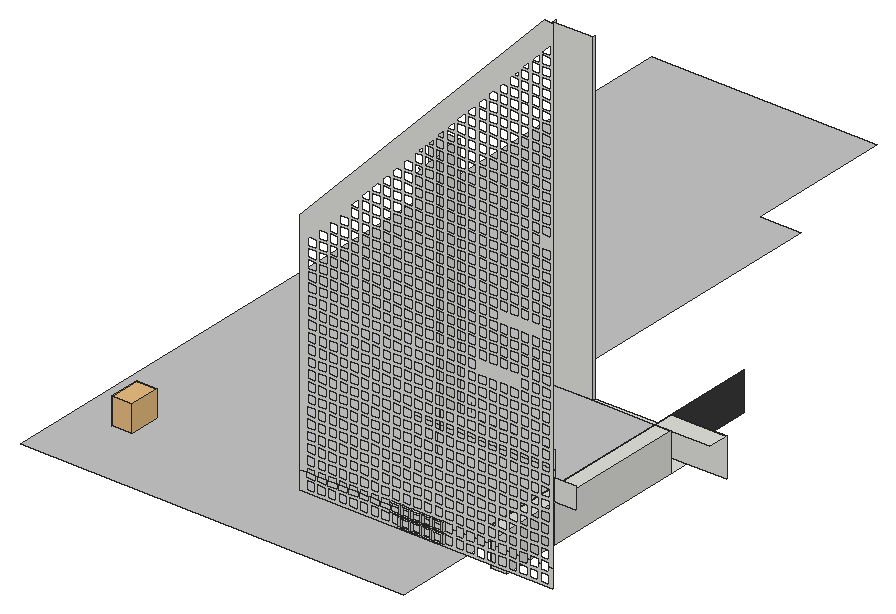
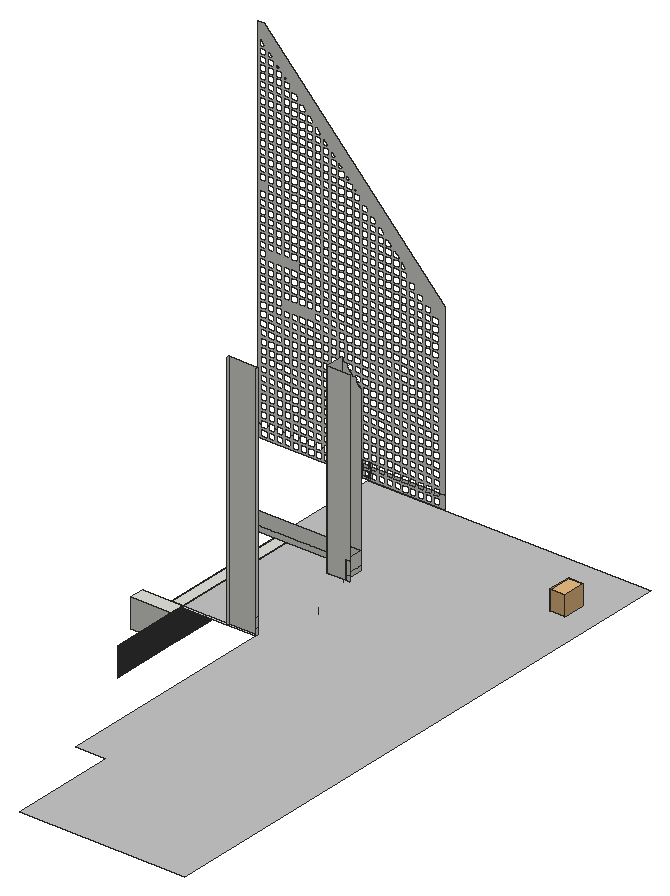
# SketchUp Ruby script. Lengths in inches.
U = 1.inch
M = Sketchup.active_model
def pt(a) = Geom::Point3d.new(a.map { |v| v * U })
def face(e, loops, mat)
  f = e.add_face(loops[0].map { |a| pt(a) })
  loops[1..].each { |l| e.add_face(l.map { |a| pt(a) }).erase! }
  f.material = f.back_material = mat if mat
  f
end
# faces: each face lists its corners as indices into pts; further lists are holes
def faces(e, pts, list, mat = nil) = list.each { |f| face(e, (f[0].is_a?(Array) ? f : [f]).map { |l| l.map { |i| pts[i] } }, mat) }
# xy, xz, yz: faces in a plane at the given z, y or x. An outline is a flat list of corners, or four numbers for a rectangle; further outlines are holes
def ring(l) = l.size == 4 ? [[l[0], l[1]], [l[2], l[1]], [l[2], l[3]], [l[0], l[3]]] : l.each_slice(2).to_a
def flat(e, list, mat, &to3) = list.each { |f| face(e, (f[0].is_a?(Array) ? f : [f]).map { |l| ring(l).map { |u, v| to3.(u, v) } }, mat) }
def xy(e, z, list, mat = nil) = flat(e, list, mat) { |x, y| [x, y, z] }
def xz(e, y, list, mat = nil) = flat(e, list, mat) { |x, z| [x, y, z] }
def yz(e, x, list, mat = nil) = flat(e, list, mat) { |y, z| [x, y, z] }
def lines(e, pts, list) = list.each { |a, b| e.add_line(pt(pts[a]), pt(pts[b])) }
# prism: a flat outline (further loops are holes) pulled along v
def prism(e, loops, v, mat = nil)
  f = face(e, loops, mat); d = Geom::Vector3d.new(v.map { |x| x * U })
  f.pushpull(f.normal.samedirection?(d) ? d.length : -d.length)
end
def box(e, o, s, mat = nil) = prism(e, [[o, [o[0] + s[0], o[1], o[2]], [o[0] + s[0], o[1] + s[1], o[2]], [o[0], o[1] + s[1], o[2]]]], [0, 0, s[2]], mat)
def at(x, y, z, deg = 0) = Geom::Transformation.translation(pt([x, y, z])) * Geom::Transformation.rotation(ORIGIN, Z_AXIS, deg.degrees)
def axes(o, x, y, z) = Geom::Transformation.new([*x, 0, *y, 0, *z, 0, *pt(o).to_a, 1])
def part(name) = M.definitions.add(name)
# library, detail: a bought-in or finely detailed component or shape, given as its bounding box
def library(name, o, s) = part(name).tap { |d| box(d.entities, o, s) }
def detail(e, o, s) = box(e.add_group.entities, o, s)
def put(e, d, t, mat = nil) = e.add_instance(d, t).tap { |i| i.material = mat if mat }
def group(e, t, mat = nil) = e.add_group.tap { |g| g.transformation = t; g.material = mat if mat }.entities
root = M.entities
M.materials.add("[Color M02]").color = [198, 198, 198]
M.materials.add("[Color M07]").color = [58, 58, 58]
c1 = library("Group\#13",[0,0,0],[3.54,3.54,3.9375])
xy(root,240.47,[[463.64,505.3125,468.02,561.375],[463.64,561.375,468.02,567.01]])
xy(root,251.0625,[[463.64,505.3125,468.02,561.375],[435.78,561.375,446.59,562.32],[446.59,561.375,463.64,562.32],[463.64,561.375,478.78,567.01]])
xy(root,251.0625,[[363.02,469.875,363.02,686.3125,424.39,686.3125,424.39,646.3125,435.78,646.3125,435.78,561.375,463.64,561.375,463.64,505.3125,468.02,505.3125,468.02,469.875]],"[Color M02]")
xy(root,257.0625,[[429.58,521.5625,435.78,528.48],[435.78,521.5625,436.5,528.48]])
xy(root,259.68,[[458.94,480.14,461.25,480.77],[461.85,480.14,464.17,480.77],[464.77,480.14,467.08,480.77],[467.68,480.14,469.99,480.77]])
xy(root,262,[[458.94,480.14,461.25,480.77],[461.85,480.14,464.17,480.77],[464.77,480.14,467.08,480.77],[467.68,480.14,469.99,480.77]])
xy(root,262.73,[[456.06,480.14,458.37,480.77],[458.97,480.14,461.28,480.77],[461.88,480.14,464.2,480.77],[464.8,480.14,467.11,480.77],[467.71,480.14,470.02,480.77]])
xy(root,265.04,[[456.06,480.14,458.37,480.77],[458.97,480.14,461.28,480.77],[461.88,480.14,464.2,480.77],[464.8,480.14,467.11,480.77],[467.71,480.14,470.02,480.77]])
xz(root,480.77,[[[430.97,258.95,430.97,263.89,432.76,263.89,432.76,262.73,435.08,262.73,435.08,263.89,435.68,263.89,435.68,262.73,437.99,262.73,437.99,263.89,438.59,263.89,438.59,262.73,440.9,262.73,440.9,263.89,441.5,263.89,441.5,262.73,443.8125,262.73,443.8125,263.89,444.41,263.89,444.41,262.73,446.72,262.73,446.72,263.89,447.32,263.89,447.32,262.73,449.64,262.73,449.64,263.89,450.24,263.89,450.24,262.73,452.55,262.73,452.55,263.89,453.15,263.89,453.15,262.73,455.46,262.73,455.46,263.89,456.06,263.89,456.06,262.73,458.37,262.73,458.37,263.89,458.97,263.89,458.97,262.73,461.28,262.73,461.28,263.89,461.88,263.89,461.88,262.73,464.2,262.73,464.2,263.89,464.8,263.89,464.8,262.73,467.11,262.73,467.11,263.89,467.71,263.89,467.71,262.73,470.02,262.73,470.02,263.89,470.62,263.89,470.62,262.73,472.93,262.73,472.93,263.89,473.53,263.89,473.53,262.73,475.84,262.73,475.84,263.89,476.44,263.89,476.44,262.73,478.76,262.73,478.76,263.89,479.36,263.89,479.36,262.73,481.67,262.73,481.67,263.89,482.27,263.89,482.27,262.73,484.58,262.73,484.58,263.89,485.18,263.89,485.18,262.73,487.49,262.73,487.49,263.89,488.09,263.89,488.09,262.73,490.4,262.73,490.4,263.89,491,263.89,491,262.73,493.32,262.73,493.32,263.89,493.92,263.89,493.92,262.73,496.23,262.73,496.23,263.89,496.83,263.89,496.83,262.73,499.14,262.73,499.14,263.89,500.29,263.89,500.29,258.95],[496.8,259.68,499.11,262],[493.89,259.68,496.2,262],[490.97,259.68,493.29,262],[488.0625,259.68,490.375,262],[485.15,259.68,487.46,262],[482.24,259.68,484.55,262],[479.33,259.68,481.64,262],[476.41,259.68,478.73,262],[473.5,259.68,475.81,262],[470.59,259.68,472.9,262],[467.68,259.68,469.99,262],[464.77,259.68,467.08,262],[461.85,259.68,464.17,262],[458.94,259.68,461.25,262],[456.03,259.68,458.34,262],[453.12,259.68,455.43,262],[450.21,259.68,452.52,262],[447.29,259.68,449.61,262],[444.38,259.68,446.69,262],[441.47,259.68,443.78,262],[438.56,259.68,440.87,262],[435.65,259.68,437.96,262],[432.73,259.68,435.05,262]],[432.76,262.73,435.08,263.89],[435.68,262.73,437.99,263.89],[438.59,262.73,440.9,263.89],[441.5,262.73,443.8125,263.89],
  [444.41,262.73,446.72,263.89],[447.32,262.73,449.64,263.89],[450.24,262.73,452.55,263.89],[453.15,262.73,455.46,263.89],[456.06,262.73,458.37,263.89],
  [458.97,262.73,461.28,263.89],[461.88,262.73,464.2,263.89],[464.8,262.73,467.11,263.89],[467.71,262.73,470.02,263.89],[[430.97,263.89,430.97,326.5,498.04,397.75,500.29,397.75,500.29,263.89,499.14,263.89,499.14,265.04,496.83,265.04,496.83,263.89,496.23,263.89,496.23,265.04,493.92,265.04,493.92,263.89,493.32,263.89,493.32,265.04,491,265.04,491,263.89,490.4,263.89,490.4,265.04,488.09,265.04,488.09,263.89,487.49,263.89,487.49,265.04,485.18,265.04,485.18,263.89,484.58,263.89,484.58,265.04,482.27,265.04,482.27,263.89,481.67,263.89,481.67,265.04,479.36,265.04,479.36,263.89,478.76,263.89,478.76,265.04,476.44,265.04,476.44,263.89,475.84,263.89,475.84,265.04,473.53,265.04,473.53,263.89,472.93,263.89,472.93,265.04,470.62,265.04,470.62,263.89,470.02,263.89,470.02,265.04,467.71,265.04,467.71,263.89,467.11,263.89,467.11,265.04,464.8,265.04,464.8,263.89,464.2,263.89,464.2,265.04,461.88,265.04,461.88,263.89,461.28,263.89,461.28,265.04,458.97,265.04,458.97,263.89,458.37,263.89,458.37,265.04,456.06,265.04,456.06,263.89,455.46,263.89,455.46,265.04,453.15,265.04,453.15,263.89,452.55,263.89,452.55,265.04,450.24,265.04,450.24,263.89,449.64,263.89,449.64,265.04,447.32,265.04,447.32,263.89,446.72,263.89,446.72,265.04,444.41,265.04,444.41,263.89,443.8125,263.89,443.8125,265.04,441.5,265.04,441.5,263.89,440.9,263.89,440.9,265.04,438.59,265.04,438.59,263.89,437.99,263.89,437.99,265.04,435.68,265.04,435.68,263.89,435.08,263.89,435.08,265.04,432.76,265.04,432.76,263.89],[485.59,370.27,487.93,372.59],[497.26,386.84,499.58,389.15],[497.26,384.09,499.58,386.4],[494.35,384.09,496.66,386.4],[494.33,381.34,496.64,383.65],[497.26,381.34,499.58,383.65],[497.26,378.59,499.58,380.9],[494.33,378.59,496.64,380.9],[491.41,375.84,493.73,378.15],[494.35,375.84,496.66,378.15],[497.26,375.84,499.58,378.15],[497.26,373.09,499.58,375.4],[494.33,373.09,496.64,375.4],[491.4375,373.09,493.75,375.4],[488.5,373.09,490.8125,375.4],[494.33,370.27,496.64,372.59],[497.26,370.27,499.58,372.59],[488.53,370.27,490.84,372.59],[482.7,370.27,485.02,372.59],[479.79,367.46,482.1,369.77],[482.7,367.46,485.02,369.77],[485.61,367.46,487.93,369.77],[488.53,367.46,490.84,369.77],[491.4375,367.46,493.75,369.77],[494.35,367.46,496.66,369.77],[497.26,367.46,499.58,369.77],[497.26,364.65,499.58,366.96],[494.35,364.65,496.66,366.96],[491.4375,364.65,493.75,366.96],[488.53,364.65,490.84,366.96],[485.61,364.65,487.93,366.96],[482.7,364.65,485.02,366.96],[479.79,364.65,482.1,366.96],[476.88,364.65,479.19,366.96],[473.97,361.84,476.28,364.15],[476.88,361.84,479.19,364.15],[479.79,361.84,482.1,364.15],[482.7,361.84,485.02,364.15],[485.61,361.84,487.93,364.15],[488.53,361.84,490.84,364.15],[491.4375,361.84,493.75,364.15],[494.35,361.84,496.66,364.15],[497.26,361.84,499.58,364.15],[497.26,359.02,499.58,361.34],[494.35,359.02,496.66,361.34],[491.4375,359.02,493.75,361.34],[488.53,359.02,490.84,361.34],[485.61,359.02,487.93,361.34],[482.7,359.02,485.02,361.34],[479.79,359.02,482.1,361.34],[476.88,359.02,479.19,361.34],[473.97,359.02,476.28,361.34],[471.05,359.02,473.37,361.34],[468.14,356.21,470.45,358.52],[471.05,356.21,473.37,358.52],[473.97,356.21,476.28,358.52],[476.88,356.21,479.19,358.52],[479.79,356.21,482.1,358.52],[482.7,356.21,485.02,358.52],[485.61,356.21,487.93,358.52],[488.53,356.21,490.84,358.52],[491.4375,356.21,493.75,358.52],[494.35,356.21,496.66,358.52],[497.26,356.21,499.58,358.52],[465.23,350.59,467.54,352.9],[468.14,353.4,470.45,355.71],[468.14,350.59,470.45,352.9],[471.05,350.59,473.37,352.9],[471.05,353.4,473.37,355.71],[473.97,353.4,476.28,355.71],[473.97,350.59,476.28,352.9],[476.88,353.4,479.19,355.71],[476.88,350.59,479.19,352.9],[479.79,353.4,482.1,355.71],[479.79,350.59,482.1,352.9],[482.7,353.4,485.02,355.71],[482.7,350.59,485.02,352.9],[485.61,353.4,487.93,355.71],[485.61,350.59,487.93,352.9],[488.53,350.59,490.84,352.9],[488.53,353.4,490.84,355.71],[491.4375,353.4,493.75,355.71],[494.35,353.4,496.66,355.71],[497.26,353.4,499.58,355.71],[497.26,350.59,499.58,352.9],[494.35,350.59,496.66,352.9],[491.4375,350.59,493.75,352.9],[497.26,347.77,499.58,350.09],[494.35,347.77,496.66,350.09],[491.4375,347.77,493.75,350.09],[488.53,347.77,490.84,350.09],[485.61,347.77,487.93,350.09],[482.7,347.77,485.02,350.09],[479.79,347.77,482.1,350.09],[476.88,347.77,479.19,350.09],[473.97,347.77,476.28,350.09],[471.05,347.77,473.37,350.09],[468.14,347.77,470.45,350.09],[465.23,347.77,467.54,350.09],[462.32,347.77,464.63,350.09],[459.41,344.96,461.72,347.27],[462.32,344.96,464.63,347.27],[465.23,344.96,467.54,347.27],[468.14,344.96,470.45,347.27],[471.05,344.96,473.37,347.27],[473.97,344.96,476.28,347.27],[476.88,344.96,479.19,347.27],[479.79,344.96,482.1,347.27],[482.7,344.96,485.02,347.27],[485.61,344.96,487.93,347.27],[488.53,344.96,490.84,347.27],[491.4375,344.96,493.75,347.27],[494.35,344.96,496.66,347.27],[497.26,344.96,499.58,347.27],[450.67,336.52,452.98,338.84],[453.58,336.52,455.89,338.84],[456.49,336.52,458.81,338.84],[459.41,336.52,461.72,338.84],[462.32,336.52,464.63,338.84],[465.23,336.52,467.54,338.84],[468.14,336.52,470.45,338.84],[471.05,336.52,473.37,338.84],[473.97,336.52,476.28,338.84],[476.88,336.52,479.19,338.84],[476.88,339.34,479.19,341.65],[473.97,339.34,476.28,341.65],[471.05,339.34,473.37,341.65],[468.14,339.34,470.45,341.65],[465.23,339.34,467.54,341.65],[462.32,339.34,464.63,341.65],[459.41,339.34,461.72,341.65],[456.49,339.34,458.81,341.65],[453.58,339.34,455.89,341.65],[456.49,342.15,458.81,344.46],[459.41,342.15,461.72,344.46],[462.32,342.15,464.63,344.46],[465.23,342.15,467.54,344.46],[468.14,342.15,470.45,344.46],[471.05,342.15,473.37,344.46],[473.97,342.15,476.28,344.46],[476.88,342.15,479.19,344.46],[479.79,342.15,482.1,344.46],[479.79,339.34,482.1,341.65],[479.79,336.52,482.1,338.84],[482.7,336.52,485.02,338.84],[482.7,339.34,485.02,341.65],[482.7,342.15,485.02,344.46],[485.61,342.15,487.93,344.46],[485.61,339.34,487.93,341.65],[485.61,336.52,487.93,338.84],[488.53,336.52,490.84,338.84],[488.53,339.34,490.84,341.65],[488.53,342.15,490.84,344.46],[491.4375,342.15,493.75,344.46],[491.4375,339.34,493.75,341.65],[491.4375,336.52,493.75,338.84],[494.35,336.52,496.66,338.84],[494.35,339.34,496.66,341.65],[494.35,342.15,496.66,344.46],[497.26,339.34,499.58,341.65],[497.26,336.52,499.58,338.84],[497.26,333.71,499.58,336.02],[494.35,333.71,496.66,336.02],[491.4375,333.71,493.75,336.02],[488.53,333.71,490.84,336.02],[485.61,333.71,487.93,336.02],[482.7,333.71,485.02,336.02],[479.79,333.71,482.1,336.02],[476.88,333.71,479.19,336.02],[473.97,333.71,476.28,336.02],[471.05,333.71,473.37,336.02],[468.14,333.71,470.45,336.02],[465.23,333.71,467.54,336.02],[462.32,333.71,464.63,336.02],[459.41,333.71,461.72,336.02],[456.49,333.71,458.81,336.02],[453.58,333.71,455.89,336.02],[450.67,333.71,452.98,336.02],[447.76,333.71,450.07,336.02],[444.85,330.9,447.16,333.21],[447.76,330.9,450.07,333.21],[450.67,330.9,452.98,333.21],[453.58,330.9,455.89,333.21],[456.49,330.9,458.81,333.21],[459.41,330.9,461.72,333.21],[462.32,330.9,464.63,333.21],[465.23,330.9,467.54,333.21],[468.14,330.9,470.45,333.21],[471.05,330.9,473.37,333.21],[473.97,330.9,476.28,333.21],[476.88,330.9,479.19,333.21],[479.79,330.9,482.1,333.21],[482.7,330.9,485.02,333.21],[485.61,330.9,487.93,333.21],[488.53,330.9,490.84,333.21],[491.4375,330.9,493.75,333.21],[494.35,330.9,496.66,333.21],[497.26,330.9,499.58,333.21],[497.26,328.09,499.58,330.4],[494.35,328.09,496.66,330.4],[491.4375,328.09,493.75,330.4],[488.53,328.09,490.84,330.4],[485.61,328.09,487.93,330.4],[482.7,328.09,485.02,330.4],[479.79,328.09,482.1,330.4],[476.88,328.09,479.19,330.4],[473.97,328.09,476.28,330.4],[471.05,328.09,473.37,330.4],[468.14,328.09,470.45,330.4],[465.23,328.09,467.54,330.4],[462.32,328.09,464.63,330.4],[459.41,328.09,461.72,330.4],[456.49,328.09,458.81,330.4],[453.58,328.09,455.89,330.4],[450.67,328.09,452.98,330.4],[447.76,328.09,450.07,330.4],[444.85,328.09,447.16,330.4],[441.93,328.09,444.25,330.4],[439.02,325.27,441.33,327.59],[441.93,325.27,444.25,327.59],[444.85,325.27,447.16,327.59],[447.76,325.27,450.07,327.59],[450.67,325.27,452.98,327.59],[453.58,325.27,455.89,327.59],[456.49,325.27,458.81,327.59],[459.41,325.27,461.72,327.59],[462.32,325.27,464.63,327.59],[465.23,325.27,467.54,327.59],[468.14,325.27,470.45,327.59],[471.05,325.27,473.37,327.59],[473.97,325.27,476.28,327.59],[476.88,325.27,479.19,327.59],[479.79,325.27,482.1,327.59],[482.7,325.27,485.02,327.59],[485.61,325.27,487.93,327.59],[488.53,325.27,490.84,327.59],[491.4375,325.27,493.75,327.59],[494.35,325.27,496.66,327.59],[497.26,325.27,499.58,327.59],[497.26,322.46,499.58,324.77],[494.35,322.46,496.66,324.77],[491.4375,322.46,493.75,324.77],[488.53,322.46,490.84,324.77],[485.61,322.46,487.93,324.77],[482.7,322.46,485.02,324.77],[479.79,322.46,482.1,324.77],[476.88,322.46,479.19,324.77],[473.97,322.46,476.28,324.77],[471.05,322.46,473.37,324.77],[468.14,322.46,470.45,324.77],[465.23,322.46,467.54,324.77],[462.32,322.46,464.63,324.77],[459.41,322.46,461.72,324.77],[459.41,319.65,461.72,321.96],[462.32,319.65,464.63,321.96],[465.23,319.65,467.54,321.96],[468.14,319.65,470.45,321.96],[471.05,319.65,473.37,321.96],[473.97,319.65,476.28,321.96],[476.88,319.65,479.19,321.96],[479.79,319.65,482.1,321.96],[482.7,319.65,485.02,321.96],[497.26,319.65,499.58,321.96],[497.26,316.84,499.58,319.15],[494.35,316.84,496.66,319.15],[491.4375,316.84,493.75,319.15],[488.53,316.84,490.84,319.15],[485.61,316.84,487.93,319.15],[482.7,316.84,485.02,319.15],[479.79,316.84,482.1,319.15],[476.88,316.84,479.19,319.15],[473.97,316.84,476.28,319.15],[471.05,316.84,473.37,319.15],[468.14,316.84,470.45,319.15],[465.23,316.84,467.54,319.15],[462.32,316.84,464.63,319.15],[459.41,316.84,461.72,319.15],[459.41,314.02,461.72,316.34],[462.32,314.02,464.63,316.34],[465.23,314.02,467.54,316.34],[468.14,314.02,470.45,316.34],[471.05,314.02,473.37,316.34],[473.97,314.02,476.28,316.34],[476.88,314.02,479.19,316.34],[479.79,314.02,482.1,316.34],[482.7,314.02,485.02,316.34],[485.61,314.02,487.93,316.34],[488.53,314.02,490.84,316.34],[491.4375,314.02,493.75,316.34],[494.35,314.02,496.66,316.34],[497.26,314.02,499.58,316.34],[439.02,322.46,441.33,324.77],[441.93,322.46,444.25,324.77],[444.85,322.46,447.16,324.77],[447.76,322.46,450.07,324.77],[450.67,322.46,452.98,324.77],[453.58,322.46,455.89,324.77],[456.49,322.46,458.81,324.77],[456.49,319.65,458.81,321.96],[456.49,316.84,458.81,319.15],[456.49,314.02,458.81,316.34],[453.58,314.02,455.89,316.34],[453.58,316.84,455.89,319.15],[453.58,319.65,455.89,321.96],[450.67,319.65,452.98,321.96],[447.76,319.65,450.07,321.96],[444.85,319.65,447.16,321.96],[441.93,319.65,444.25,321.96],[439.02,319.65,441.33,321.96],[436.11,319.65,438.42,321.96],[433.2,316.84,435.51,319.15],[436.11,316.84,438.42,319.15],[439.02,316.84,441.33,319.15],[441.93,316.84,444.25,319.15],[444.85,316.84,447.16,319.15],[447.76,316.84,450.07,319.15],[450.67,316.84,452.98,319.15],[450.67,314.02,452.98,316.34],[447.76,314.02,450.07,316.34],[444.85,314.02,447.16,316.34],[441.93,314.02,444.25,316.34],[439.02,314.02,441.33,316.34],[436.11,314.02,438.42,316.34],[433.2,314.02,435.51,316.34],[433.2,311.21,435.51,313.52],[436.11,311.21,438.42,313.52],[439.02,311.21,441.33,313.52],[441.93,311.21,444.25,313.52],[444.85,311.21,447.16,313.52],[447.76,311.21,450.07,313.52],[450.67,311.21,452.98,313.52],[453.58,311.21,455.89,313.52],[456.49,311.21,458.81,313.52],[459.41,311.21,461.72,313.52],[462.32,311.21,464.63,313.52],[465.23,311.21,467.54,313.52],[468.14,311.21,470.45,313.52],[471.05,311.21,473.37,313.52],[473.97,311.21,476.28,313.52],[476.88,311.21,479.19,313.52],[479.79,311.21,482.1,313.52],[482.7,311.21,485.02,313.52],[485.61,311.21,487.93,313.52],[488.53,311.21,490.84,313.52],[491.4375,311.21,493.75,313.52],[494.35,311.21,496.66,313.52],[497.26,311.21,499.58,313.52],[433.2,308.4,435.51,310.71],[436.11,308.4,438.42,310.71],[439.02,308.4,441.33,310.71],[441.93,308.4,444.25,310.71],[444.85,308.4,447.16,310.71],[447.76,308.4,450.07,310.71],[450.67,308.4,452.98,310.71],[453.58,308.4,455.89,310.71],[456.49,308.4,458.81,310.71],[459.41,308.4,461.72,310.71],[462.32,308.4,464.63,310.71],[465.23,308.4,467.54,310.71],[468.14,308.4,470.45,310.71],[471.05,308.4,473.37,310.71],[473.97,308.4,476.28,310.71],[476.88,308.4,479.19,310.71],[479.79,308.4,482.1,310.71],[482.7,308.4,485.02,310.71],[485.61,308.4,487.93,310.71],[488.53,308.4,490.84,310.71],[491.4375,308.4,493.75,310.71],[494.35,308.4,496.66,310.71],[497.26,308.4,499.58,310.71],[497.23,305.35,499.55,307.67],[494.32,305.35,496.63,307.67],[491.41,305.35,493.72,307.67],[476.85,305.35,479.16,307.67],[473.9375,305.35,476.25,307.67],[471.03,305.35,473.34,307.67],[468.11,305.35,470.43,307.67],[465.2,305.35,467.51,307.67],[462.29,305.35,464.6,307.67],[459.38,305.35,461.69,307.67],[456.47,305.35,458.78,307.67],[453.55,305.35,455.87,307.67],[450.64,305.35,452.95,307.67],[447.73,305.35,450.04,307.67],[444.82,305.35,447.13,307.67],[441.91,305.35,444.22,307.67],[438.99,305.35,441.31,307.67],[436.08,305.35,438.39,307.67],[433.17,305.35,435.48,307.67],[433.14,302.31,435.45,304.62],[436.05,302.31,438.36,304.62],[438.96,302.31,441.28,304.62],[441.875,302.31,444.1875,304.62],[444.79,302.31,447.1,304.62],[447.7,302.31,450.01,304.62],[450.61,302.31,452.92,304.62],[453.52,302.31,455.84,304.62],[456.4375,302.31,458.75,304.62],[459.35,302.31,461.66,304.62],[462.26,302.31,464.57,304.62],[465.17,302.31,467.48,304.62],[468.08,302.31,470.4,304.62],[471,302.31,473.31,304.62],[473.91,302.31,476.22,304.62],[476.82,302.31,479.13,304.62],[479.73,302.31,482.04,304.62],[482.64,302.31,484.96,304.62],[485.56,302.31,487.87,304.62],[488.47,302.31,490.78,304.62],[491.38,302.31,493.69,304.62],[494.29,302.31,496.61,304.62],[497.2,302.31,499.52,304.62],[497.18,299.27,499.49,301.58],[494.26,299.27,496.58,301.58],[491.35,299.27,493.66,301.58],[488.44,299.27,490.75,301.58],[485.53,299.27,487.84,301.58],[482.62,299.27,484.93,301.58],[479.7,299.27,482.02,301.58],[476.79,299.27,479.1,301.58],[473.88,299.27,476.19,301.58],[470.97,299.27,473.28,301.58],[468.06,299.27,470.37,301.58],[465.14,299.27,467.46,301.58],[462.23,299.27,464.54,301.58],[459.32,299.27,461.63,301.58],[456.41,299.27,458.72,301.58],[453.5,299.27,455.81,301.58],[450.58,299.27,452.9,301.58],[447.67,299.27,449.98,301.58],[444.76,299.27,447.07,301.58],[441.85,299.27,444.16,301.58],[438.93,299.27,441.25,301.58],[436.02,299.27,438.34,301.58],[433.11,299.27,435.42,301.58],[433.08,296.22,435.39,298.53],[435.99,296.22,438.31,298.53],[438.91,296.22,441.22,298.53],[441.82,296.22,444.13,298.53],[444.73,296.22,447.04,298.53],[447.64,296.22,449.95,298.53],[450.55,296.22,452.87,298.53],[453.47,296.22,455.78,298.53],[456.38,296.22,458.69,298.53],[459.29,296.22,461.6,298.53],[462.2,296.22,464.51,298.53],[465.11,296.22,467.43,298.53],[468.03,296.22,470.34,298.53],[470.9375,296.22,473.25,298.53],[473.85,296.22,476.16,298.53],[476.76,296.22,479.07,298.53],[479.67,296.22,481.99,298.53],[482.59,296.22,484.9,298.53],[485.5,296.22,487.8125,298.53],[488.41,296.22,490.72,298.53],[491.32,296.22,493.64,298.53],[494.23,296.22,496.55,298.53],[497.15,296.22,499.46,298.53],[433.05,293.18,435.37,295.49],[435.96,293.18,438.28,295.49],[438.875,293.18,441.1875,295.49],[441.79,293.18,444.1,295.49],[444.7,293.18,447.01,295.49],[447.61,293.18,449.93,295.49],[450.53,293.18,452.84,295.49],[453.4375,293.18,455.75,295.49],[456.35,293.18,458.66,295.49],[459.26,293.18,461.57,295.49],[462.17,293.18,464.49,295.49],[465.09,293.18,467.4,295.49],[468,293.18,470.31,295.49],[470.91,293.18,473.22,295.49],[473.82,293.18,476.13,295.49],[476.73,293.18,479.05,295.49],[479.65,293.18,481.96,295.49],[482.56,293.18,484.87,295.49],[485.47,293.18,487.78,295.49],[488.38,293.18,490.69,295.49],[491.29,293.18,493.61,295.49],[494.21,293.18,496.52,295.49],[497.12,293.18,499.43,295.49],[444.67,290.13,446.98,292.44],[447.58,290.13,449.9,292.44],[450.5,290.13,452.81,292.44],[453.41,290.13,455.72,292.44],[456.32,290.13,458.63,292.44],[459.23,290.13,461.54,292.44],[462.14,290.13,464.46,292.44],[465.06,290.13,467.37,292.44],[467.97,290.13,470.28,292.44],[470.88,290.13,473.19,292.44],[473.79,290.13,476.1,292.44],[476.7,290.13,479.02,292.44],[479.62,290.13,481.93,292.44],[482.53,290.13,484.84,292.44],[485.44,290.13,487.75,292.44],[488.35,290.13,490.67,292.44],[491.26,290.13,493.58,292.44],[494.18,290.13,496.49,292.44],[497.09,290.13,499.4,292.44],[497.06,287.09,499.37,289.4],[494.15,287.09,496.46,289.4],[491.24,287.09,493.55,289.4],[488.32,287.09,490.64,289.4],[485.41,287.09,487.72,289.4],[482.5,287.09,484.8125,289.4],[479.59,287.09,481.9,289.4],[476.68,287.09,478.99,289.4],[473.76,287.09,476.08,289.4],[470.85,287.09,473.16,289.4],[467.9375,287.09,470.25,289.4],[465.03,287.09,467.34,289.4],[462.12,287.09,464.43,289.4],[459.2,287.09,461.52,289.4],[456.29,287.09,458.6,289.4],[453.38,287.09,455.69,289.4],[450.47,287.09,452.78,289.4],[447.56,287.09,449.87,289.4],[444.64,287.09,446.96,289.4],[444.61,284.04,446.93,286.35],[447.53,284.04,449.84,286.35],[450.4375,284.04,452.75,286.35],[453.35,284.04,455.66,286.35],[456.26,284.04,458.57,286.35],[459.17,284.04,461.49,286.35],[462.09,284.04,464.4,286.35],[465,284.04,467.3125,286.35],[467.91,284.04,470.22,286.35],[470.82,284.04,473.13,286.35],[473.73,284.04,476.05,286.35],[476.65,284.04,478.96,286.35],[479.56,284.04,481.87,286.35],[482.47,284.04,484.78,286.35],[485.38,284.04,487.7,286.35],[488.29,284.04,490.61,286.35],[491.21,284.04,493.52,286.35],[494.12,284.04,496.43,286.35],[497.03,284.04,499.34,286.35],[497,281,499.3125,283.31],[494.09,281,496.4,283.31],[491.18,281,493.49,283.31],[488.27,281,490.58,283.31],[485.35,281,487.67,283.31],[482.44,281,484.75,283.31],[479.53,281,481.84,283.31],[476.62,281,478.93,283.31],[473.71,281,476.02,283.31],[470.79,281,473.11,283.31],[467.88,281,470.19,283.31],[464.97,281,467.28,283.31],[462.06,281,464.37,283.31],[459.15,281,461.46,283.31],[456.23,281,458.55,283.31],[453.32,281,455.63,283.31],[450.41,281,452.72,283.31],[447.5,281,449.81,283.31],[447.47,277.95,449.78,280.26],[450.38,277.95,452.69,280.26],[453.29,277.95,455.6,280.26],[456.2,277.95,458.52,280.26],[459.12,277.95,461.43,280.26],[462.03,277.95,464.34,280.26],[464.94,277.95,467.25,280.26],[467.85,277.95,470.16,280.26],[470.76,277.95,473.08,280.26],[473.68,277.95,475.99,280.26],[476.59,277.95,478.9,280.26],[479.5,277.95,481.8125,280.26],[482.41,277.95,484.73,280.26],[485.32,277.95,487.64,280.26],[488.24,277.95,490.55,280.26],[491.15,277.95,493.46,280.26],[494.0625,277.95,496.375,280.26],[496.97,277.95,499.29,280.26],[496.94,274.91,499.26,277.22],[494.03,274.91,496.34,277.22],[491.12,274.91,493.43,277.22],[488.21,274.91,490.52,277.22],[485.3,274.91,487.61,277.22],[482.38,274.91,484.7,277.22],[479.47,274.91,481.78,277.22],[476.56,274.91,478.87,277.22],[473.65,274.91,475.96,277.22],[470.74,274.91,473.05,277.22],[467.82,274.91,470.14,277.22],[464.91,274.91,467.22,277.22],[462,274.91,464.3125,277.22],[459.09,274.91,461.4,277.22],[456.18,274.91,458.49,277.22],[453.26,274.91,455.58,277.22],[450.35,274.91,452.66,277.22],[447.4375,274.91,449.75,277.22],[444.59,281,446.9,283.31],[444.56,277.95,446.87,280.26],[444.53,274.91,446.84,277.22],[441.62,274.91,443.93,277.22],[441.64,277.95,443.96,280.26],[441.67,281,443.99,283.31],[441.7,284.04,444.01,286.35],[441.73,287.09,444.04,289.4],[441.76,290.13,444.07,292.44],[438.85,290.13,441.16,292.44],[438.82,287.09,441.13,289.4],[438.79,284.04,441.1,286.35],[438.76,281,441.07,283.31],[435.82,277.95,438.13,280.26],[438.73,277.95,441.04,280.26],[438.7,274.91,441.02,277.22],[435.79,274.91,438.1,277.22],[435.85,281,438.16,283.31],[435.88,284.04,438.19,286.35],[435.91,287.09,438.22,289.4],[435.9375,290.13,438.25,292.44],[433.02,290.13,435.34,292.44],[432.99,287.09,435.31,289.4],[432.97,284.04,435.28,286.35],[432.9375,281,435.25,283.31],[432.91,277.95,435.22,280.26],[432.88,274.91,435.19,277.22],[432.85,271.86,435.16,274.17],[435.76,271.86,438.07,274.17],[438.67,271.86,440.99,274.17],[441.59,271.86,443.9,274.17],[444.5,271.86,446.8125,274.17],[447.41,271.86,449.72,274.17],[450.32,271.86,452.63,274.17],[453.23,271.86,455.55,274.17],[456.15,271.86,458.46,274.17],[459.06,271.86,461.37,274.17],[461.97,271.86,464.28,274.17],[464.88,271.86,467.19,274.17],[467.79,271.86,470.11,274.17],[470.71,271.86,473.02,274.17],[473.62,271.86,475.93,274.17],[476.53,271.86,478.84,274.17],[479.44,271.86,481.76,274.17],[482.35,271.86,484.67,274.17],[485.27,271.86,487.58,274.17],[488.18,271.86,490.49,274.17],[491.09,271.86,493.4,274.17],[494,271.86,496.32,274.17],[496.91,271.86,499.23,274.17],[496.89,268.82,499.2,271.13],[493.97,268.82,496.29,271.13],[491.0625,268.82,493.375,271.13],[488.15,268.82,490.46,271.13],[485.24,268.82,487.55,271.13],[482.33,268.82,484.64,271.13],[479.41,268.82,481.73,271.13],[476.5,268.82,478.8125,271.13],[473.59,268.82,475.9,271.13],[470.68,268.82,472.99,271.13],[467.77,268.82,470.08,271.13],[464.85,268.82,467.17,271.13],[461.94,268.82,464.25,271.13],[459.03,268.82,461.34,271.13],[456.12,268.82,458.43,271.13],[453.21,268.82,455.52,271.13],[450.29,268.82,452.61,271.13],[447.38,268.82,449.69,271.13],[444.47,268.82,446.78,271.13],[441.56,268.82,443.87,271.13],[438.65,268.82,440.96,271.13],[435.73,268.82,438.05,271.13],[432.82,268.82,435.13,271.13],[432.79,265.77,435.1,268.09],[435.7,265.77,438.02,268.09],[438.62,265.77,440.93,268.09],[441.53,265.77,443.84,268.09],[444.44,265.77,446.75,268.09],[447.35,265.77,449.66,268.09],[450.26,265.77,452.58,268.09],[453.18,265.77,455.49,268.09],[456.09,265.77,458.4,268.09],[459,265.77,461.3125,268.09],[461.91,265.77,464.22,268.09],[464.82,265.77,467.14,268.09],[467.74,265.77,470.05,268.09],[470.65,265.77,472.96,268.09],[473.56,265.77,475.87,268.09],[476.47,265.77,478.79,268.09],[479.38,265.77,481.7,268.09],[482.3,265.77,484.61,268.09],[485.21,265.77,487.52,268.09],[488.12,265.77,490.43,268.09],[491.03,265.77,493.35,268.09],[493.94,265.77,496.26,268.09],[496.86,265.77,499.17,268.09],[491.4375,381.34,493.75,381.34,493.75,383.65,491.55,383.65,491.4375,383.53],[491.4375,378.59,493.75,378.59,493.75,380.9,491.55,380.9,491.4375,380.78],[488.53,375.84,490.84,375.84,490.84,378.15,488.64,378.15,488.53,378.03],[485.61,373.09,487.93,373.09,487.93,375.4,485.72,375.4,485.61,375.28],[491.4375,370.27,493.75,370.27,493.75,372.59,491.55,372.59,491.4375,372.47],[465.23,353.4,467.54,353.4,467.54,355.71,465.36,355.71,465.23,355.57],[436.11,322.46,438.42,322.46,438.42,324.77,436.37,324.77,436.11,324.5],[462.32,350.59,464.63,350.59,464.63,352.9,462.73,352.9,462.32,352.46],[488.53,378.59,490.84,378.59,490.84,380.9,488.97,380.9,488.53,380.43],[433.2,319.65,435.51,319.65,435.51,321.96,433.73,321.96,433.2,321.39],[459.41,347.77,461.72,347.77,461.72,350.09,460.09,350.09,459.41,349.36],[485.61,375.84,487.93,375.84,487.93,378.15,486.39,378.15,485.61,377.32],[456.49,344.96,458.81,344.96,458.81,347.27,457.45,347.27,456.49,346.25],[482.7,373.09,485.02,373.09,485.02,375.4,483.82,375.4,482.7,374.21],[453.58,342.15,455.89,342.15,455.89,344.46,454.82,344.46,453.58,343.14],[479.79,370.27,482.1,370.27,482.1,372.59,481.18,372.59,479.79,371.11],[450.67,339.34,452.98,339.34,452.98,341.65,452.18,341.65,450.67,340.04],[476.88,367.46,479.19,367.46,479.19,369.77,478.54,369.77,476.88,368],[447.76,336.52,450.07,336.52,450.07,338.84,449.55,338.84,447.76,336.93],[473.97,364.65,476.28,364.65,476.28,366.96,475.91,366.96,473.97,364.89],[497.26,389.59,499.58,389.59,499.58,391.9,499.28,391.9,497.26,389.75],[444.85,333.71,447.16,333.71,447.16,336.02,446.91,336.02,444.85,333.82],[471.1,361.84,473.37,361.84,473.37,364.15,473.27,364.15],[494.54,386.84,496.66,386.84,496.66,389.11],[468.47,359.02,470.45,359.02,470.45,361.14],[491.96,384.09,493.75,384.09,493.75,386],[465.83,356.21,467.54,356.21,467.54,358.04],[489.38,381.34,490.84,381.34,490.84,382.89],[463.19,353.4,464.63,353.4,464.63,354.93]]])
xz(root,505.3125,[[463.64,240.47,468.02,251.0625]])
xz(root,521.5625,[[468.02,251.0625,473.73,257.0625],[429.58,257.0625,436.5,258.95],[436.5,257.0625,468.02,258.95],[429.58,258.95,436.5,263.89],[436.5,258.95,468.02,263.89],
  [429.58,263.89,436.5,263.89,436.5,325.17,435.5625,324.17,435.11,324.6,434.23,323.67,434.68,323.24,432.26,320.67,431.81,321.1,430.93,320.17,431.39,319.74,430.04,318.3,429.58,317.82]])
xz(root,528.48,[[428,257.0625,429.58,258.95],[429.58,257.0625,436.5,257.0625,436.5,326.08,428,326.08,428,263.89,429.58,263.89],[428,258.95,429.58,263.89]])
xz(root,561.375,[[463.64,240.47,468.02,251.0625],[435.78,251.0625,446.59,340.125]])
xz(root,567.01,[[463.64,240.47,478.78,251.0625]])
yz(root,429.58,[[521.5625,257.0625,528.48,258.95],[521.5625,258.95,528.48,263.89]])
yz(root,435.78,[[561.375,251.0625,562.32,253.4375],[561.375,253.4375,562.32,257.0625],[561.375,257.0625,562.32,340.125]])
yz(root,436.5,[[521.5625,257.0625,528.48,326.08]])
yz(root,446.59,[[561.375,251.0625,562.32,340.125]])
yz(root,458.34,[[480.14,259.68,480.77,262]])
yz(root,458.37,[[480.14,262.73,480.77,265.04]])
yz(root,458.94,[[480.14,259.68,480.77,262]])
yz(root,458.97,[[480.14,262.73,480.77,265.04]])
yz(root,461.25,[[480.14,259.68,480.77,262]])
yz(root,461.28,[[480.14,262.73,480.77,265.04]])
yz(root,461.85,[[480.14,259.68,480.77,262]])
yz(root,461.88,[[480.14,262.73,480.77,265.04]])
yz(root,463.64,[[505.3125,240.47,561.375,251.0625],[561.375,240.47,567.01,251.0625],[567.01,240.47,591.8125,251.0625]],"[Color M07]")
yz(root,464.17,[[480.14,259.68,480.77,262]])
yz(root,464.2,[[480.14,262.73,480.77,265.04]])
yz(root,464.77,[[480.14,259.68,480.77,262]])
yz(root,464.8,[[480.14,262.73,480.77,265.04]])
yz(root,467.08,[[480.14,259.68,480.77,262]])
yz(root,467.11,[[480.14,262.73,480.77,265.04]])
yz(root,467.68,[[480.14,259.68,480.77,262]])
yz(root,467.71,[[480.14,262.73,480.77,265.04]])
yz(root,468.02,[[505.3125,240.47,521.5625,251.0625],[521.5625,240.47,561.375,251.0625]])
yz(root,469.99,[[480.14,259.68,480.77,262]])
yz(root,470.02,[[480.14,262.73,480.77,265.04]])
yz(root,470.59,[[480.14,259.68,480.77,262]])
yz(root,470.62,[[480.14,262.73,480.77,265.04]])
p = [[429.58,541.0625,251.0625],[429.58,541.0625,253.4375],[435.78,521.5625,251.0625],[435.78,521.5625,257.0625],[435.78,561.375,240.47],[435.78,562.32,240.47],
  [429.58,561.375,240.47]]
lines(root,p,[[0,1],[2,3],[4,5],[6,4]])
put(root,c1,axes([378.57,488.625,258.17],[-1.5535,0,0],[0,2.39,0],[0,0,-3.63878]))
